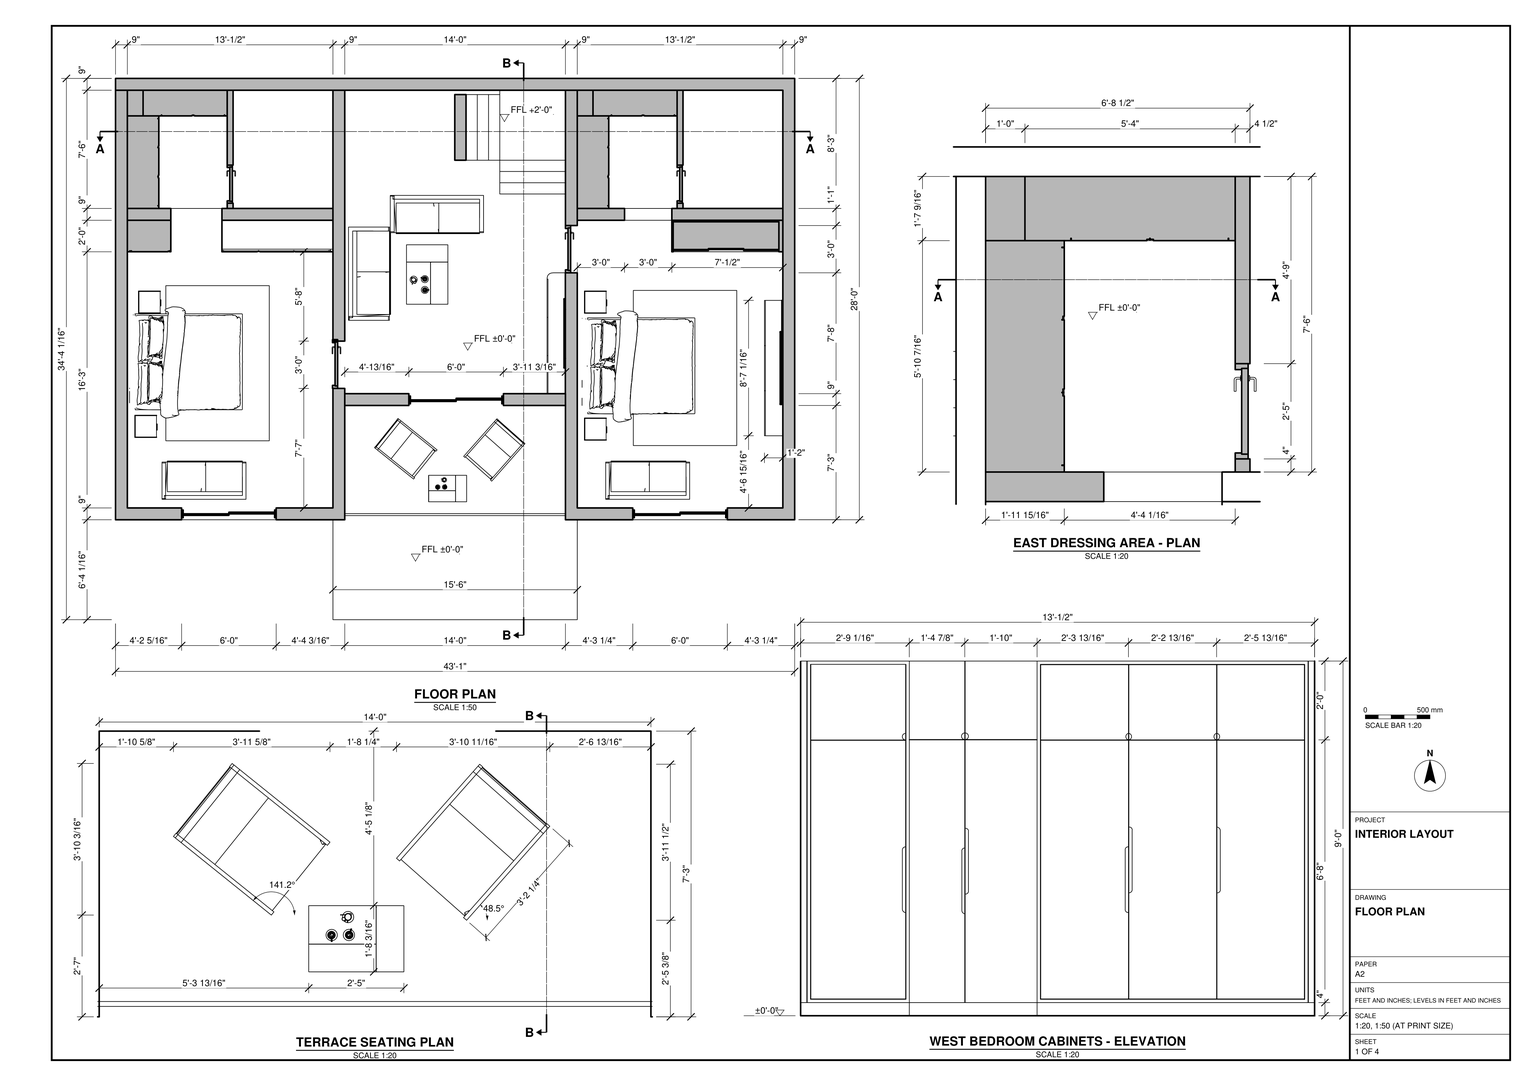
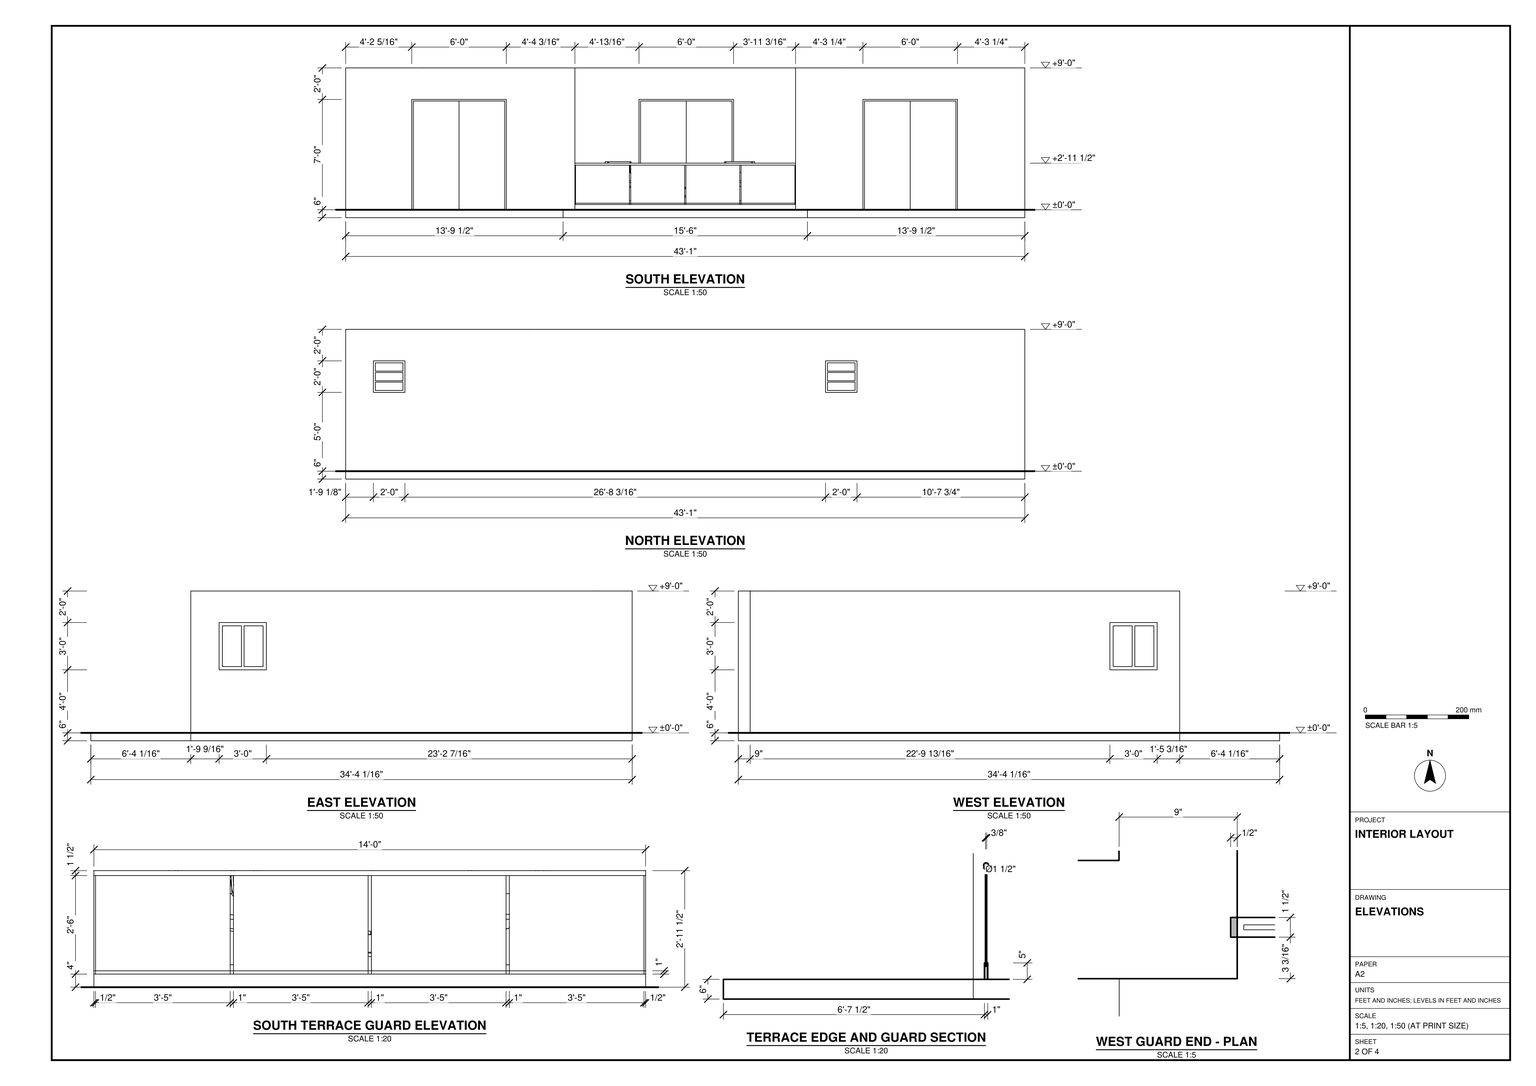
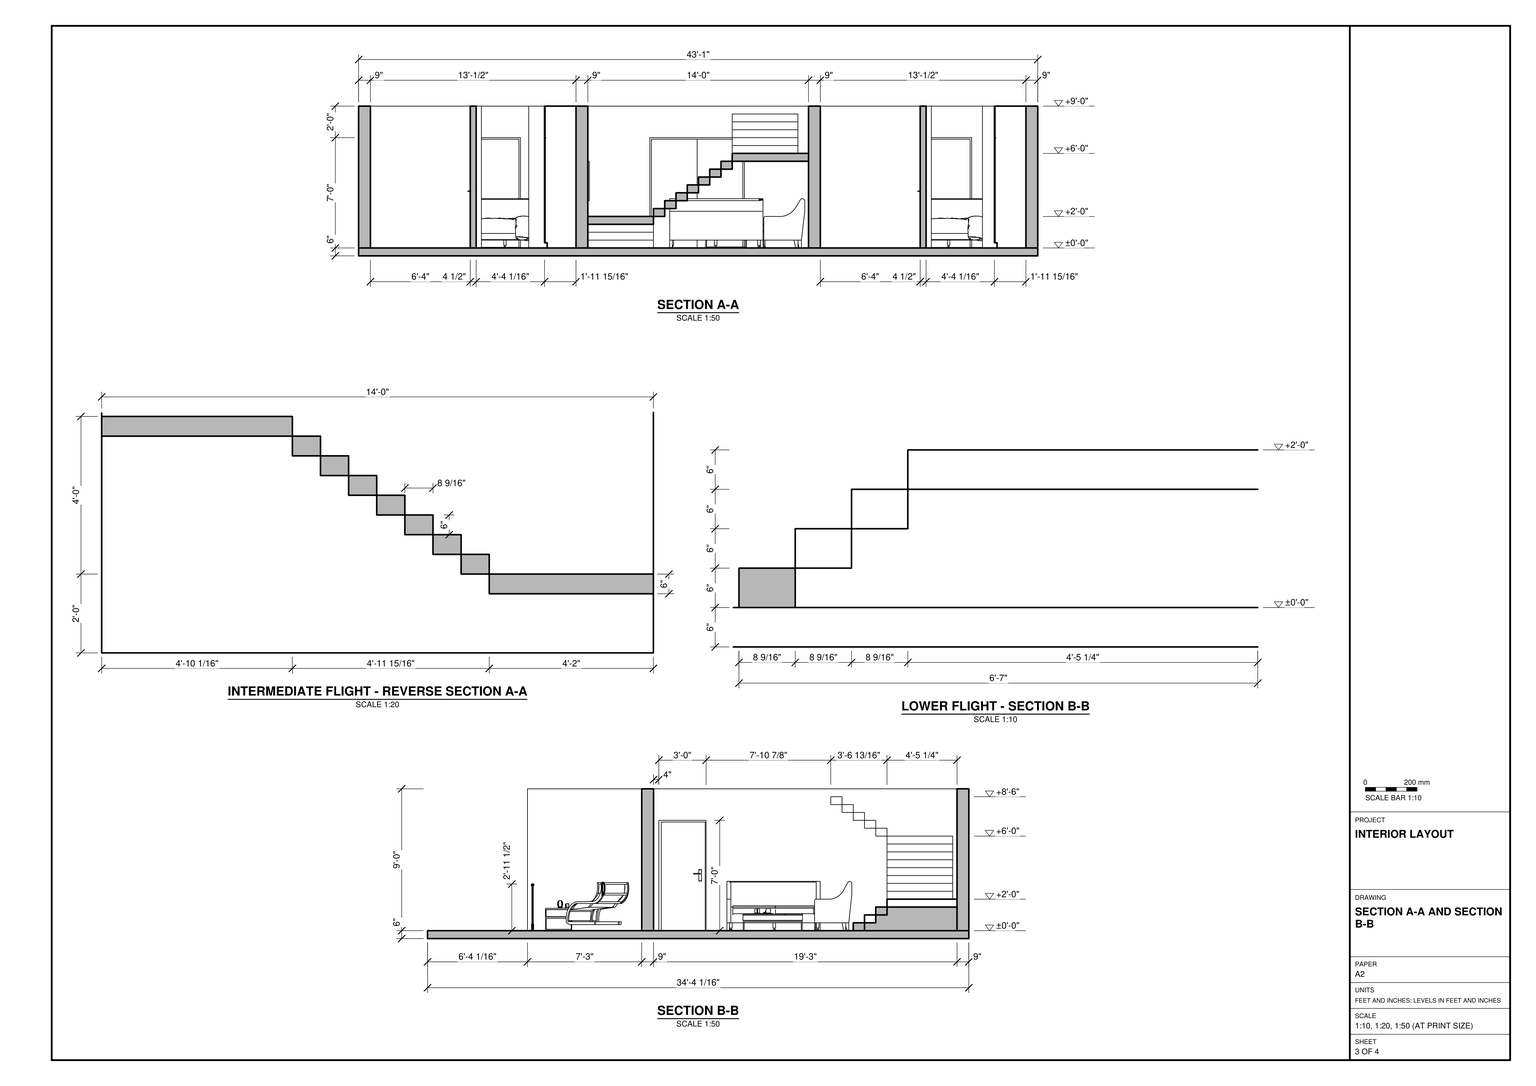
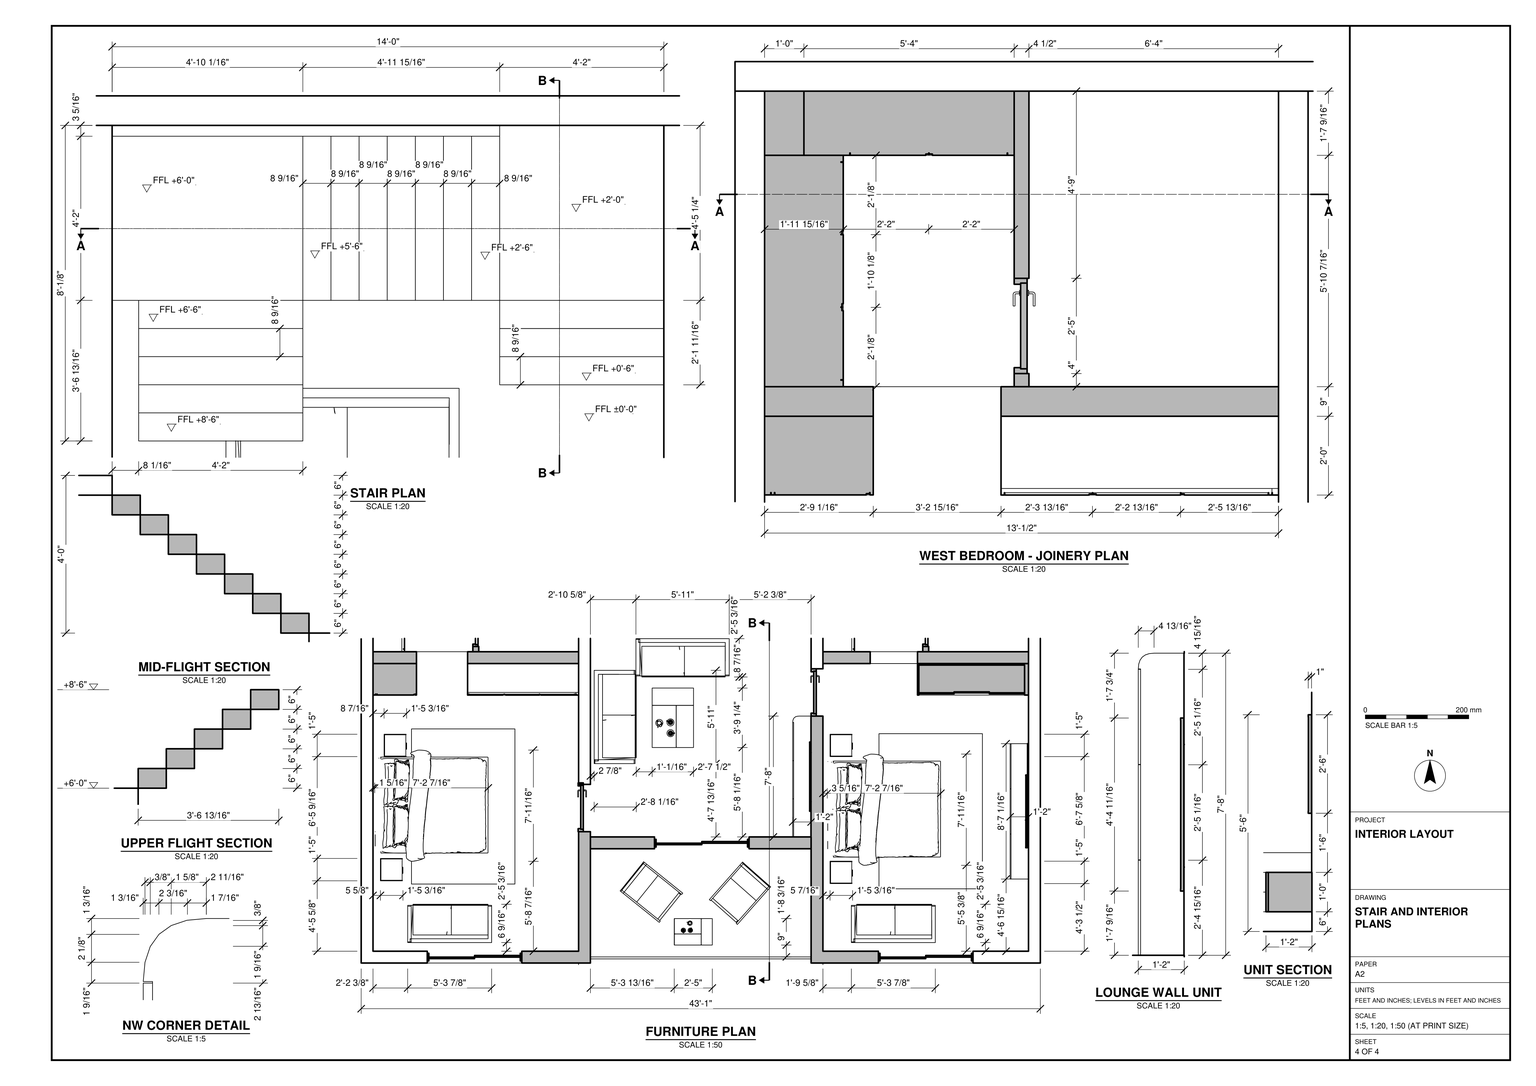
Build the furnished interior in SketchUp from task_files/diagram_01.pdf. Work in feet and inches. The overall model extents are 51'-9 7/16" along X, 51'-6" along Y and 9'-6" along Z. Set the finished floor at ±0'-0". Use the 43'-1" width on the south elevation to lay out the shell rather than stretching the rooms to the overall model width.

Place the west and east bedrooms on either side of the central lounge, with dressing areas to the north and a recessed seating terrace to the south. Model the 6" floor slab, the 9" perimeter and main dividing walls, and the thinner partitions at their drawn thicknesses. Follow the elevations for the framed south openings, the high north windows and the windows in the side walls. Use the sections to build the turning stair at the north end of the lounge, including its flights and landings. Fit the terrace guard between the bedroom wings.

Model the dressing-area storage and the west bedroom cabinet fronts. Match the footprints and orientations of the beds, bedside tables, bedroom seating, lounge sofas, low tables and terrace chairs to the plan. Decor and loose items may be any suitable library components. Keep shell elements and individual furniture and joinery pieces in separate groups or components, and use components for repeated parts. Save one SketchUp model as output_files/two_bedroom_interior_with_a_central_lounge_and_terrace.skp.

# SketchUp Ruby script. Lengths in inches.
U = 1.inch
M = Sketchup.active_model
def pt(a) = Geom::Point3d.new(a.map { |v| v * U })
def face(e, loops, mat)
  f = e.add_face(loops[0].map { |a| pt(a) })
  loops[1..].each { |l| e.add_face(l.map { |a| pt(a) }).erase! }
  f.material = f.back_material = mat if mat
  f
end
# faces: each face lists its corners as indices into pts; further lists are holes
def faces(e, pts, list, mat = nil) = list.each { |f| face(e, (f[0].is_a?(Array) ? f : [f]).map { |l| l.map { |i| pts[i] } }, mat) }
# xy, xz, yz: faces in a plane at the given z, y or x. An outline is a flat list of corners, or four numbers for a rectangle; further outlines are holes
def ring(l) = l.size == 4 ? [[l[0], l[1]], [l[2], l[1]], [l[2], l[3]], [l[0], l[3]]] : l.each_slice(2).to_a
def flat(e, list, mat, &to3) = list.each { |f| face(e, (f[0].is_a?(Array) ? f : [f]).map { |l| ring(l).map { |u, v| to3.(u, v) } }, mat) }
def xy(e, z, list, mat = nil) = flat(e, list, mat) { |x, y| [x, y, z] }
def xz(e, y, list, mat = nil) = flat(e, list, mat) { |x, z| [x, y, z] }
def yz(e, x, list, mat = nil) = flat(e, list, mat) { |y, z| [x, y, z] }
def lines(e, pts, list) = list.each { |a, b| e.add_line(pt(pts[a]), pt(pts[b])) }
# prism: a flat outline (further loops are holes) pulled along v
def prism(e, loops, v, mat = nil)
  f = face(e, loops, mat); d = Geom::Vector3d.new(v.map { |x| x * U })
  f.pushpull(f.normal.samedirection?(d) ? d.length : -d.length)
end
def box(e, o, s, mat = nil) = prism(e, [[o, [o[0] + s[0], o[1], o[2]], [o[0] + s[0], o[1] + s[1], o[2]], [o[0], o[1] + s[1], o[2]]]], [0, 0, s[2]], mat)
def at(x, y, z, deg = 0) = Geom::Transformation.translation(pt([x, y, z])) * Geom::Transformation.rotation(ORIGIN, Z_AXIS, deg.degrees)
def axes(o, x, y, z) = Geom::Transformation.new([*x, 0, *y, 0, *z, 0, *pt(o).to_a, 1])
def part(name) = M.definitions.add(name)
# library, detail: a bought-in or finely detailed component or shape, given as its bounding box
def library(name, o, s) = part(name).tap { |d| box(d.entities, o, s) }
def detail(e, o, s) = box(e.add_group.entities, o, s)
def put(e, d, t, mat = nil) = e.add_instance(d, t).tap { |i| i.material = mat if mat }
def group(e, t, mat = nil) = e.add_group.tap { |g| g.transformation = t; g.material = mat if mat }.entities
root = M.entities
M.materials.add("0555 AP 9271 HERBAL GREEN").color = [64, 196, 176]
M.materials.add("0899 AP 7833 SUNKISSED").color = [249, 236, 185]
M.materials.add("DDR840RVS01100X").color = [126, 127, 125]
M.materials.add("Glass Railing Color").color = [198, 198, 198]
M.materials.add("Railing Glass").color = [63, 150, 137]
M.materials["Railing Glass"].alpha = 0.13
M.materials.add("Travertine (WDB2F6)").color = [204, 197, 184]
M.materials.add("[0136_Charcoal]").color = [35, 35, 35]
M.materials.add("[Color M09]").color = [0, 0, 0]
M.materials.add("[Translucent Glass Blue]").color = [100, 149, 237]
M.materials["[Translucent Glass Blue]"].alpha = 0.5
M.materials.add("[Translucent Glass Gray]").color = [128, 128, 128]
M.materials["[Translucent Glass Gray]"].alpha = 0.5
M.materials.add("[Wood Bamboo]").color = [177, 105, 43]
c1 = part("Tall decorative panel")
xy(c1.entities,0,[[0,0,26.83,0.71]])
xy(c1.entities,102,[[0,0,26.83,0.71]])
xz(c1.entities,0,[[0,51,26.83,102]],"0555 AP 9271 HERBAL GREEN")
xz(c1.entities,0,[[0,0,26.83,51]],"0899 AP 7833 SUNKISSED")
xz(c1.entities,0.71,[[0,0,26.83,102]])
yz(c1.entities,0,[[0,0,0.71,102]])
yz(c1.entities,26.83,[[0,0,0.71,102]])
c2 = library("SOFA",[-1,-71,-0.18],[36,71,37.74])
c3 = library("Спалня Венид",[0.07,-0.07,0],[84.71,86.8,39])
c4 = part("Handle Detail - Push Button Lock")
detail(c4.entities,[0,0,0],[0.6875,0.39,0.6875])
c5 = library("Sofa_Table H32xW80xL115",[-5.98,-0.08,0],[45.27,31.5,16.9375])
c6 = library("Untitled",[0,-0.2,0],[24.17,23.98,23.92])
c7 = part("Carpet v15 (4)")
xy(c7.entities,0,[[-70.87,0,47.24,78.74]])
xy(c7.entities,0.39,[[-70.87,0,47.24,78.74]],"DDR840RVS01100X")
xz(c7.entities,0,[[-70.87,0,47.24,0.39]])
xz(c7.entities,78.74,[[-70.87,0,47.24,0.39]])
yz(c7.entities,-70.87,[[0,0,78.74,0.39]])
yz(c7.entities,47.24,[[0,0,78.74,0.39]])
c8 = library("Untitled\#1",[2.47,0,4.63],[38.23,28.5,32])
c9 = library("Group145\#1",[-18,-45,0],[35.91,90,0.71])
c10 = part("Group12\#1")
xy(c10.entities,0,[[465.75,76.08,465.75,85.08,508,85.08,508,403.08,0,403.08,0,412.08,517,412.08,517,76.08],[342.5,76.08,342.5,264.08,351.5,264.08,351.5,85.08,393.75,85.08,393.75,76.08],[342.5,300.08,351.5,403.08]])
xy(c10.entities,18,[[342.42,172.08,342.5,198.88],[342.42,199,342.5,236.22],[342.42,236.33,342.5,264.08]])
xy(c10.entities,48,[[508,97.64,517,133.64]])
xy(c10.entities,60,[[127.73,403.08,151.73,412.08],[471.9,403.08,495.9,412.08]])
xy(c10.entities,84,[[393.75,76.08,465.75,85.08],[508,97.64,517,133.64],[342.5,264.08,351.5,300.08],[127.73,403.08,151.73,412.08],[471.9,403.08,495.9,412.08]])
xy(c10.entities,108,[[342.5,76.08,517,76.08,517,412.08,0,412.08,0,403.08,508,403.08,508,85.08,351.5,85.08,351.5,403.08,342.5,403.08,342.5,264.08,342.42,264.08,342.42,236.33,342.5,236.33,342.5,236.22,342.42,236.22,342.42,199,342.5,199,342.5,198.88,342.42,198.88,342.42,172.08,342.5,172.08]])
xz(c10.entities,76.08,[[342.5,0,393.75,0,393.75,84,465.75,84,465.75,0,517,0,517,108,342.5,108]])
xz(c10.entities,85.08,[[351.5,0,351.5,108,508,108,508,0,465.75,0,465.75,84,393.75,84,393.75,0]])
xz(c10.entities,97.64,[[508,48,517,84]])
xz(c10.entities,133.64,[[508,48,517,84]])
xz(c10.entities,172.08,[[342.42,18,342.5,108]])
xz(c10.entities,198.88,[[342.42,18,342.5,108]])
xz(c10.entities,199,[[342.42,18,342.5,108]])
xz(c10.entities,236.22,[[342.42,18,342.5,108]])
xz(c10.entities,236.33,[[342.42,18,342.5,108]])
xz(c10.entities,264.08,[[342.5,0,342.5,18,342.42,18,342.42,84,351.5,84,351.5,0],[342.42,84,342.5,108]])
xz(c10.entities,300.08,[[342.5,0,351.5,84]])
xz(c10.entities,403.08,[[[0,0,342.5,108],[127.73,60,151.73,84]],[342.5,0,351.5,108],[[351.5,0,508,108],[471.9,60,495.9,84]]])
xz(c10.entities,412.08,[[[0,0,517,108],[127.73,60,151.73,84],[471.9,60,495.9,84]]])
yz(c10.entities,0,[[403.08,0,412.08,108]])
yz(c10.entities,127.73,[[403.08,60,412.08,84]])
yz(c10.entities,151.73,[[403.08,60,412.08,84]])
yz(c10.entities,342.42,[[172.08,18,198.88,108],[199,18,236.22,108],[236.33,18,264.08,108]])
yz(c10.entities,342.5,[[76.08,0,76.08,108,172.08,108,172.08,18,264.08,18,264.08,0],[300.08,0,300.08,84,264.2,84,264.2,108,403.08,108,403.08,0],[198.88,18,199,108],[236.22,18,236.33,108],[264.08,84,264.2,108]])
yz(c10.entities,351.5,[[85.08,0,264.08,0,264.08,84,300.08,84,300.08,0,403.08,0,403.08,108,85.08,108]])
yz(c10.entities,393.75,[[76.08,0,85.08,84]])
yz(c10.entities,465.75,[[76.08,0,85.08,84]])
yz(c10.entities,471.9,[[403.08,60,412.08,84]])
yz(c10.entities,495.9,[[403.08,60,412.08,84]])
yz(c10.entities,508,[[[85.08,0,85.08,108,140.03,108,140.03,18,243.09,18,243.09,108,403.08,108,403.08,0],[97.64,48,133.64,84]],[140.03,18,207.09,108],[207.09,18,243.09,108]])
yz(c10.entities,517,[[[76.08,0,412.08,108],[97.64,48,133.64,84]]])
put(c10.entities,c9,axes([508,225.09,63],[0,-1,0],[0,0,1],[-1,0,0]),"[Wood Bamboo]")
c11 = part("Group15\#1")
xy(c11.entities,0,[[0,76.08,0,403.08,9,403.08,9,85.08,50.29,85.08,50.29,76.08],[122.29,76.08,122.29,85.08,165.5,85.08,165.5,176.08,174.5,176.08,174.5,76.08],[165.5,212.08,174.5,403.08]])
xy(c11.entities,48,[[0,93.26,9,129.26]])
xy(c11.entities,84,[[50.29,76.08,122.29,85.08],[0,93.26,9,129.26],[165.5,176.08,174.5,212.08]])
xy(c11.entities,108,[[0,76.08,174.5,76.08,174.5,403.08,165.5,403.08,165.5,85.08,9,85.08,9,403.08,0,403.08]])
xz(c11.entities,76.08,[[0,0,50.29,0,50.29,84,122.29,84,122.29,0,174.5,0,174.5,108,0,108]])
xz(c11.entities,85.08,[[9,0,9,108,165.5,108,165.5,0,122.29,0,122.29,84,50.29,84,50.29,0]])
xz(c11.entities,93.26,[[0,48,9,84]])
xz(c11.entities,129.26,[[0,48,9,84]])
xz(c11.entities,176.08,[[165.5,0,174.5,84]])
xz(c11.entities,212.08,[[165.5,0,174.5,84]])
xz(c11.entities,403.08,[[0,0,9,108],[165.5,0,174.5,108]])
yz(c11.entities,0,[[[76.08,0,403.08,108],[93.26,48,129.26,84]]])
yz(c11.entities,9,[[[85.08,0,403.08,108],[93.26,48,129.26,84]]])
yz(c11.entities,50.29,[[76.08,0,85.08,84]])
yz(c11.entities,122.29,[[76.08,0,85.08,84]])
yz(c11.entities,165.5,[[85.08,0,85.08,108,403.08,108,403.08,0,212.08,0,212.08,84,176.08,84,176.08,0]])
yz(c11.entities,174.5,[[76.08,0,176.08,0,176.08,84,212.08,84,212.08,0,403.08,0,403.08,108,76.08,108]])
c12 = part("Group16\#1")
prism(c12.entities,[[[342.5,172.08,0],[295.29,172.08,0],[295.29,172.08,84],[223.29,172.08,84],[223.29,172.08,0],[174.5,172.08,0],[174.5,172.08,108],[342.5,172.08,108]]],[0,-9,0])
c13 = part("Group17\#1")
box(c13.entities,[81,304.08,0],[84.5,9,108])
box(c13.entities,[9,304.08,0],[33.09,9,108])
p = [[81,313.08,0],[42.09,313.08,0]]
lines(c13.entities,p,[[0,1]])
c14 = part("Group18\#1")
xy(c14.entities,0,[[351.5,304.08,387.49,313.08],[387.49,304.08,423.5,313.08],[423.5,304.08,508,313.08]])
xy(c14.entities,108,[[351.5,304.08,387.49,313.08],[423.5,304.08,508,313.08]])
xz(c14.entities,304.08,[[351.5,0,387.49,108],[423.5,0,508,108]])
xz(c14.entities,313.08,[[351.5,0,387.49,108],[423.5,0,508,108]])
yz(c14.entities,351.5,[[304.08,0,313.08,108]])
yz(c14.entities,387.49,[[304.08,0,313.08,108]])
yz(c14.entities,423.5,[[304.08,0,313.08,108]])
yz(c14.entities,508,[[304.08,0,313.08,108]])
c15 = part("Group19\#1")
prism(c15.entities,[[[89.5,313.08,0],[89.5,317.08,0],[89.5,317.08,84],[89.5,346.08,84],[89.5,346.08,0],[89.5,403.08,0],[89.5,403.08,108],[89.5,313.08,108]]],[-4.5,0,0])
c16 = part("Group20\#1")
prism(c16.entities,[[[432,313.08,0],[432,317.08,0],[432,317.08,84],[432,346.08,84],[432,346.08,0],[432,403.08,0],[432,403.08,108],[432,313.08,108]]],[-4.5,0,0])
c17 = part("Group22\#2")
xy(c17.entities,0,[[-15.5,-15.5,-1,15.5],[1,-15.5,15.5,15.5]])
c18 = part("Group21\#1")
prism(c18.entities,[[[18,-18,0],[-18,-18,0],[-18,18,0],[18,18,0]],[[15.5,15.5,0],[1,15.5,0],[1,-15.5,0],[15.5,-15.5,0]],[[-1,15.5,0],[-15.5,15.5,0],[-15.5,-15.5,0],[-1,-15.5,0]]],[0,0,4])
put(c18.entities,c17,at(0,0,2),"[Translucent Glass Blue]")
c19 = part("Group24\#2")
xy(c19.entities,0,[[-10.5,-10.5,10.5,-4.17],[-10.5,-3.17,10.5,3.17],[-10.5,4.17,10.5,10.5]])
c20 = part("Group23\#1")
prism(c20.entities,[[[12,12,0],[12,-12,0],[-12,-12,0],[-12,12,0]],[[10.5,-3.17,0],[10.5,3.17,0],[-10.5,3.17,0],[-10.5,-3.17,0]],[[-10.5,-4.17,0],[-10.5,-10.5,0],[10.5,-10.5,0],[10.5,-4.17,0]],[[-10.5,10.5,0],[-10.5,4.17,0],[10.5,4.17,0],[10.5,10.5,0]]],[0,0,4])
put(c20.entities,c19,at(0,0,2),"[Translucent Glass Blue]")
c21 = part("Group\#3")
box(c21.entities,[0,0,0],[49.98,8.5625,6])
c22 = part("Group28\#1")
prism(c22.entities,[[[36,42,0],[36,-42,0],[34.8125,-42,0],[34.8125,40.8125,0],[-34.8125,40.8125,0],[-34.8125,-42,0],[-36,-42,0],[-36,42,0]]],[0,0,5.875])
c23 = part("Group\#6")
g1 = group(c23.entities,at(36,2.9375,0),"[Translucent Glass Gray]")
box(g1,[0,0,0],[34.8125,1.25,82.8125])
g2 = group(c23.entities,at(1.1875,0,0),"[Translucent Glass Gray]")
box(g2,[0,1.8125,0],[34.8125,1.125,82.8125])
put(c23.entities,c22,axes([36,5.875,42],[1,0,0],[0,0,1],[0,-1,0]),"[0136_Charcoal]")
c24 = library("Group\#8",[0,0,0],[156.5,23.99,108])
c25 = library("Group\#12",[0,0,0],[25.96,70.46,108])
c26 = library("Group\#13",[0,0,0],[64.02,19.54,108.12])
c27 = part("Glass Rail Spacer")
box(c27.entities,[-0.5,-0.25,0],[1,0.5,1],"Glass Railing Color")
c28 = part("Group45\#1")
prism(c28.entities,[[[0.54,0,1.27],[0.38,0,1.39],[0.21,0,1.47],[0.01,0,1.5],[-0.18,0,1.48],[-0.37,0,1.41],[-0.52,0,1.29],[-0.64,0,1.13],[-0.72,0,0.96],[-0.75,0,0.76],[-0.73,0,0.57],[-0.66,0,0.38],[-0.54,0,0.23],[-0.38,0,0.11],[-0.21,0,0.03],[-0.01,0,0],[0.18,0,0.02],[0.37,0,0.09],[0.52,0,0.21],[0.64,0,0.37],[0.72,0,0.54],[0.75,0,0.74],[0.73,0,0.93],[0.66,0,1.12]]],[0,169,0],"Glass Railing Color")
c29 = part("Group48\#1")
prism(c29.entities,[[[0.25,0,5],[0.25,0,4],[-0.25,0,4],[-0.25,0,5],[-0.5,0,5],[-0.5,0,0],[0.5,0,0],[0.5,0,5]]],[0,169,0],"Glass Railing Color")
c30 = part("Group49\#1")
box(c30.entities,[-0.1875,0,0],[0.375,41,30],"Railing Glass")
c31 = part("Group50\#1")
box(c31.entities,[-0.1875,0,0],[0.375,41,30],"Railing Glass")
c32 = part("Group51\#1")
box(c32.entities,[-0.1875,0,0],[0.375,41,30],"Railing Glass")
c33 = part("Group52\#1")
box(c33.entities,[-0.1875,0,0],[0.375,41,30],"Railing Glass")
c34 = part("Glass Railing")
put(c34.entities,c27,at(0,0,4))
put(c34.entities,c27,at(42,0,4))
put(c34.entities,c27,at(84,0,4))
put(c34.entities,c27,at(126,0,4))
put(c34.entities,c27,at(168,0,4))
put(c34.entities,c28,at(-0.5,0,34,-90),"Glass Railing Color")
put(c34.entities,c29,at(-0.5,0,0,-90),"Glass Railing Color")
put(c34.entities,c30,at(0.5,0,4,-90),"Railing Glass")
put(c34.entities,c31,at(42.5,0,4,-90),"Railing Glass")
put(c34.entities,c32,at(84.5,0,4,-90),"Railing Glass")
put(c34.entities,c33,at(126.5,0,4,-90),"Railing Glass")
c35 = library("Group\#9",[0,0,0],[25.96,70.46,108])
c36 = library("Group\#10",[0,0,0],[64.02,19.54,108.12])
c37 = library("Group\#45",[0,0,0],[2.18,1.82,2.18])
c38 = library("Group\#44",[0,0,0],[2.18,1.82,2.18])
c39 = library("Group\#46",[0,0,0],[31.5,6.69,82.68])
c40 = library("Group\#47",[0,0,0],[31.5,6.69,82.68])
xy(root,108,[[9,383.55,20.98,403.08],[351.5,383.55,363.48,403.08]])
p = [[512.5,97.64,84],[512.5,97.64,48],[512.5,133.64,48],[512.5,133.64,84],[495.9,407.58,84],[495.9,407.58,60],
  [471.9,407.58,60],[471.9,407.58,84],[50.29,80.58,0],[50.29,80.58,84],[122.29,80.58,84],[122.29,80.58,0],
  [32.96,337.24,85.4375],[32.96,337.06,85.4],[32.96,336.89,85.32],[32.96,336.75,85.2],[32.96,336.64,85.05],[32.96,336.57,84.87],
  [32.96,336.55,84.6875],[32.96,336.57,84.5],[32.96,336.64,84.33],[32.96,336.75,84.18],[32.96,336.89,84.06],[32.96,337.06,83.98],
  [32.96,337.24,83.9375],[32.96,337.36,85.4375],[32.96,337.54,85.4],[32.96,337.7,85.32],[32.96,337.85,85.2],[32.96,337.95,85.05],
  [32.96,338.02,84.87],[32.96,338.04,84.6875],[32.96,338.02,84.5],[32.96,337.95,84.33],[32.96,337.85,84.18],[32.96,337.7,84.06],
  [32.96,337.54,83.98],[32.96,337.36,83.9375],[620.34,614.35,37.77],[620.47,614.35,37.77],[620.34,614.47,37.77],[620.47,614.47,37.77],
  [620.34,614.16,37.77],[620.34,613.97,37.77],[620.4,614.16,37.77],[620.22,613.97,37.77],[620.34,613.85,37.77],[620.22,613.85,37.77],
  [620.28,614.16,37.77],[620.34,613.47,37.77],[620.34,614.85,37.77]]
lines(root,p,[[0,1],[1,2],[2,3],[3,0],[4,5],[5,6],[6,7],[7,4],[8,9],[9,10],[10,11],[11,8],
  [12,13],[13,14],[14,15],[15,16],[16,17],[17,18],[18,19],[19,20],[20,21],[21,22],[22,23],[23,24],
  [25,26],[26,27],[27,28],[28,29],[29,30],[30,31],[31,32],[32,33],[33,34],[34,35],[35,36],[36,37],
  [38,39],[40,41],[42,43],[42,44],[43,45],[46,47],[42,38],[42,48],[43,46],[38,40],[46,49],[40,50]])
put(root,c1,at(424.5,281.09,5),"0555 AP 9271 HERBAL GREEN")
put(root,c1,at(451.33,281.8,5))
put(root,c1,at(478.17,281.09,5))
put(root,c2,axes([208.52,298.91,0],[-0.89,0,0],[0,1,0],[0,0,1]))
put(root,c2,axes([280.15,294.67,0],[0,0.81,0],[1,0,0],[0,0,1]))
put(root,c3,at(441.18,150.38,0,90))
put(root,c3,at(96.7,153.44,0,90))
put(root,c4,at(619.99,617.32,37.05))
put(root,c5,at(252.91,246.14,0,90))
put(root,c2,axes([437.05,120.01,0],[0,-0.81,0],[0.9,0,0],[0,0,1]))
put(root,c2,axes([99.3,120.01,0],[0,-0.81,0],[0.9,0,0],[0,0,1]))
put(root,c6,axes([356.91,233.39,0],[0.71,0,0],[0,0.71,0],[0,0,0.71]))
put(root,c6,axes([356.91,136.73,0],[0.71,0,0],[0,0.71,0],[0,0,0.71]))
put(root,c6,axes([14.625,138.82,0],[0.71,0,0],[0,0.71,0],[0,0,0.71]))
put(root,c6,axes([17.4375,233.39,0],[0.71,0,0],[0,0.71,0],[0,0,0.71]))
put(root,c7,at(117.04,207.07,0,90))
put(root,c7,at(472.91,203.45,0.11,90))
put(root,c8,at(195.19,132.5625,0,-38.8))
put(root,c8,at(292,154.85,0,-131.5))
put(root,c5,axes([242.13,89.82,0],[0.64,0,0],[0,0.64,0],[0,0,1.35475]))
g3 = group(root,at(0,76.08,-6))
xy(g3,0,[[165.51,-76.08,165.51,0,0,0,0,336,517,336,517,0,351.5,0,351.5,-76.08]])
xy(g3,6,[[165.51,-76.08,351.5,-76.08,351.5,0,517,0,517,336,0,336,0,0,165.51,0]],"Travertine (WDB2F6)")
xz(g3,-76.08,[[165.51,0,351.5,6]])
xz(g3,0,[[0,0,165.51,6],[351.5,0,517,6]])
xz(g3,336,[[0,0,517,6]])
yz(g3,0,[[0,0,336,6]])
yz(g3,165.51,[[-76.08,0,0,6]])
yz(g3,351.5,[[-76.08,0,0,6]])
yz(g3,517,[[0,0,336,6]])
put(root,c10,at(0,0,0))
put(root,c11,at(0,0,0))
put(root,c12,at(0,0,0))
put(root,c13,at(0,0,0))
put(root,c14,at(0,0,0))
put(root,c15,at(0,0,0))
put(root,c16,at(0,0,0))
put(root,c18,axes([511.625,115.64,66],[0,1,0],[0,0,1],[1,0,0]),"[Color M09]")
put(root,c18,axes([2.01,111.26,66],[0,1,0],[0,0,1],[1,0,0]),"[Color M09]")
put(root,c20,axes([483.9,407.58,72],[-1,0,0],[0,0,1],[0,1,0]),"[Color M09]")
put(root,c20,axes([139.73,406.18,72],[-1,0,0],[0,0,1],[0,1,0]),"[Color M09]")
put(root,c21,at(292.52,324.09,0))
put(root,c21,at(292.52,332.66,6))
put(root,c21,at(292.52,341.23,12))
g4 = group(root,at(292.52,349.8,18))
box(g4,[0,0,0],[49.98,53.28,6])
put(root,c21,at(292.52,349.8,24,90))
put(root,c21,at(283.95,349.8,30,90))
put(root,c21,at(275.39,349.8,36,90))
put(root,c21,at(266.83,349.8,42,90))
put(root,c21,at(258.26,349.8,48,90))
put(root,c21,at(249.7,349.8,54,90))
put(root,c21,at(241.13,349.8,60,90))
g5 = group(root,at(232.57,349.8,66,90))
box(g5,[0,0,0],[49.98,58.07,6])
put(root,c21,at(182.59,341.24,72))
put(root,c21,at(182.59,332.67,78))
put(root,c21,at(182.59,324.11,84))
put(root,c21,at(182.59,315.55,90))
put(root,c21,at(182.59,306.98,96))
put(root,c23,at(50.29,77.65,0))
put(root,c23,at(393.75,77.65,0))
put(root,c23,at(223.29,164.38,0))
g6 = group(root,at(423.5,280.09,0))
xy(g6,0,[[0,2,84.5,23.96]])
xy(g6,4,[[0,0,84.5,2]])
xy(g6,5,[[1,0,81.5,22.83]])
xy(g6,107,[[1,0,81.5,22.83]])
xy(g6,108,[[0,0,84.5,23.96]])
xz(g6,0,[[[0,4,82.5,108],[1,5,81.5,107]],[82.5,4,84.5,108]],"0555 AP 9271 HERBAL GREEN")
xz(g6,2,[[0,0,84.5,4]],"0555 AP 9271 HERBAL GREEN")
xz(g6,22.83,[[1,5,81.5,107]])
xz(g6,23.96,[[0,0,84.5,108]])
yz(g6,0,[[2,0,2,4,0,4,0,108,23.96,108,23.96,0]])
yz(g6,1,[[0,5,22.83,107]])
yz(g6,81.5,[[0,5,22.83,107]])
yz(g6,84.5,[[2,0,23.96,0,23.96,108,0,108,0,4,2,4]])
put(root,c24,at(9,280.09,0))
put(root,c25,at(9,313.08,0),"0899 AP 7833 SUNKISSED")
put(root,c26,at(20.98,383.55,0),"0899 AP 7833 SUNKISSED")
put(root,c34,at(174.5,79.99,0))
put(root,c35,at(351.5,313.08,0),"0899 AP 7833 SUNKISSED")
put(root,c36,at(363.48,383.55,0),"0899 AP 7833 SUNKISSED")
put(root,c37,at(619.25,611.16,36.3))
put(root,c38,at(621.43,618,36.3,-180))
put(root,c39,axes([164.84,213.25,0],[0,-1.18,0],[1,0,0],[0,0,1.02]))
put(root,c39,axes([342.19,300.08,0],[0,-1.143,0],[1,0,0],[0,0,1.02]))
put(root,c40,axes([427.19,346.08,0],[0,-0.92075,0],[1,0,0],[0,0,1.016]))
put(root,c40,axes([84.69,346.08,0],[0,-0.92075,0],[1,0,0],[0,0,1.016]))
g7 = group(root,at(494,140.03,6),"[Wood Bamboo]")
xy(g7,0,[[0,0,0.71,34.24],[0.71,0,14,103.0625],[0,34.35,0.71,68.59],[0,68.71,0.71,103.0625]],"[Wood Bamboo]")
xy(g7,12,[[0,0,0.71,34.24],[0.71,0,14,103.0625],[0,34.35,0.71,68.59],[0,68.71,0.71,103.0625]],"[Wood Bamboo]")
xz(g7,0,[[0,0,0.71,12],[0.71,0,14,12]],"[Wood Bamboo]")
xz(g7,34.24,[[0,0,0.71,12]],"[Wood Bamboo]")
xz(g7,34.35,[[0,0,0.71,12]],"[Wood Bamboo]")
xz(g7,68.59,[[0,0,0.71,12]],"[Wood Bamboo]")
xz(g7,68.71,[[0,0,0.71,12]],"[Wood Bamboo]")
xz(g7,103.0625,[[0,0,0.71,12],[0.71,0,14,12]],"[Wood Bamboo]")
yz(g7,0,[[0,0,34.24,12],[34.35,0,68.59,12],[68.71,0,103.0625,12]],"[Wood Bamboo]")
yz(g7,0.71,[[0,0,34.24,12],[34.24,0,34.35,12],[34.35,0,68.59,12],[68.59,0,68.71,12],[68.71,0,103.0625,12]],"[Wood Bamboo]")
yz(g7,14,[[0,0,103.0625,12]],"[Wood Bamboo]")
g8 = group(root,at(506,163.87,36),"[Color M09]")
xy(g8,0,[[-0.08,0,1,55.375]],"[Color M09]")
xy(g8,0.71,[[-0.08,0.71,0,54.67]],"[Color M09]")
xy(g8,42.29,[[-0.08,0.71,0,54.67]],"[Color M09]")
xy(g8,43,[[-0.08,0,1,55.375]],"[Color M09]")
xz(g8,0,[[-0.08,0,1,43]],"[Color M09]")
xz(g8,0.71,[[-0.08,0.71,0,42.29]],"[Color M09]")
xz(g8,54.67,[[-0.08,0.71,0,42.29]],"[Color M09]")
xz(g8,55.375,[[-0.08,0,1,43]],"[Color M09]")
yz(g8,-0.08,[[[0,0,55.375,43],[0.71,0.71,54.67,42.29]]],"[Color M09]")
yz(g8,0,[[0.71,0.71,54.67,42.29]])
yz(g8,1,[[0,0,55.375,43]],"[Color M09]")
g9 = group(root,at(328.5,172.08,6),"[Wood Bamboo]")
xy(g9,0,[[0,0,0.71,28.95],[0.71,0,0.71,87.2,0,87.2,0.13,88.67,0.53,89.87,1.2,90.8,2.13,91.47,3.33,91.87,4.8,92,14,92,14,0],[0,29.07,0.71,58.02],[0,58.13,0.71,87.08]])
xy(g9,12,[[0,0,0.71,28.95],[0.71,0,14,0,14,92,4.8,92,3.33,91.87,2.13,91.47,1.2,90.8,0.53,89.87,0.13,88.67,0,87.2,0.71,87.2],[0,29.07,0.71,58.02],[0,58.13,0.71,87.08]])
xz(g9,0,[[0,0,0.71,12],[0.71,0,14,12]])
xz(g9,28.95,[[0,0,0.71,12]])
xz(g9,29.07,[[0,0,0.71,12]])
xz(g9,58.02,[[0,0,0.71,12]])
xz(g9,58.13,[[0,0,0.71,12]])
xz(g9,87.08,[[0,0,0.71,12]])
xz(g9,87.2,[[0,0,0.71,12]])
xz(g9,92,[[4.8,0,14,12]])
yz(g9,0,[[0,0,28.95,12],[29.07,0,58.02,12],[58.13,0,87.08,12]])
yz(g9,0.71,[[0,0,28.95,12],[28.95,0,29.07,12],[29.07,0,58.02,12],[58.02,0,58.13,12],[58.13,0,87.08,12],
  [87.08,0,87.2,12]])
yz(g9,14,[[0,0,92,12]])
p = [[0,87.2,0],[0,87.2,12],[0.13,88.67,12],[0.13,88.67,0],[0.53,89.87,12],[0.53,89.87,0],
  [1.2,90.8,12],[1.2,90.8,0],[2.13,91.47,12],[2.13,91.47,0],[3.33,91.87,12],[3.33,91.87,0],
  [4.8,92,12],[4.8,92,0]]
faces(g9,p,[[0,1,2,3],[3,2,4,5],[5,4,6,7],[7,6,8,9],[9,8,10,11],[11,10,12,13]])
g10 = group(root,at(341.38,191.65,36),"[0136_Charcoal]")
xy(g10,0,[[0,0,1,52.6875]])
xy(g10,0.71,[[0,0.71,0.04,51.98]])
xy(g10,29.29,[[0,0.71,0.04,51.98]])
xy(g10,30,[[0,0,1,52.6875]])
xz(g10,0,[[0,0,1,30]])
xz(g10,0.71,[[0,0.71,0.04,29.29]])
xz(g10,51.98,[[0,0.71,0.04,29.29]])
xz(g10,52.6875,[[0,0,1,30]])
yz(g10,0,[[[0,0,52.6875,30],[0.71,0.71,51.98,29.29]]])
yz(g10,0.04,[[0.71,0.71,51.98,29.29]])
yz(g10,1,[[0,0,52.6875,30]])
